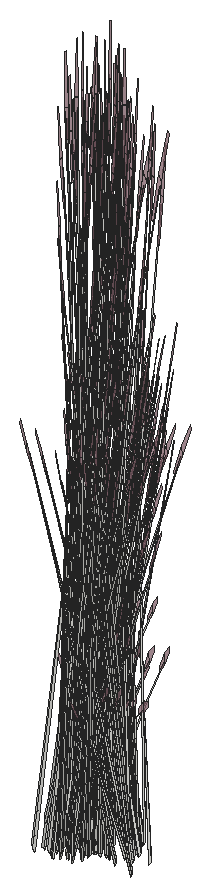
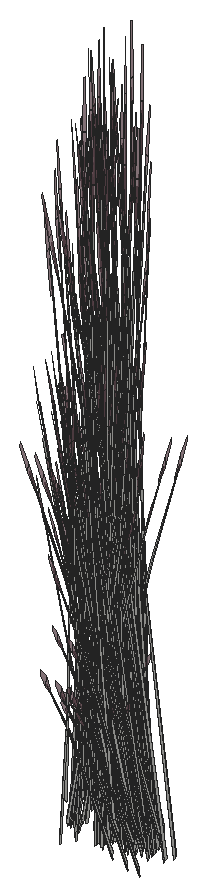
# SketchUp Ruby script. Lengths in inches.
U = 1.inch
M = Sketchup.active_model
def pt(a) = Geom::Point3d.new(a.map { |v| v * U })
def face(e, loops, mat)
  f = e.add_face(loops[0].map { |a| pt(a) })
  loops[1..].each { |l| e.add_face(l.map { |a| pt(a) }).erase! }
  f.material = f.back_material = mat if mat
  f
end
# faces: each face lists its corners as indices into pts; further lists are holes
def faces(e, pts, list, mat = nil) = list.each { |f| face(e, (f[0].is_a?(Array) ? f : [f]).map { |l| l.map { |i| pts[i] } }, mat) }
# xy, xz, yz: faces in a plane at the given z, y or x. An outline is a flat list of corners, or four numbers for a rectangle; further outlines are holes
def ring(l) = l.size == 4 ? [[l[0], l[1]], [l[2], l[1]], [l[2], l[3]], [l[0], l[3]]] : l.each_slice(2).to_a
def flat(e, list, mat, &to3) = list.each { |f| face(e, (f[0].is_a?(Array) ? f : [f]).map { |l| ring(l).map { |u, v| to3.(u, v) } }, mat) }
def xy(e, z, list, mat = nil) = flat(e, list, mat) { |x, y| [x, y, z] }
def xz(e, y, list, mat = nil) = flat(e, list, mat) { |x, z| [x, y, z] }
def yz(e, x, list, mat = nil) = flat(e, list, mat) { |y, z| [x, y, z] }
def lines(e, pts, list) = list.each { |a, b| e.add_line(pt(pts[a]), pt(pts[b])) }
# prism: a flat outline (further loops are holes) pulled along v
def prism(e, loops, v, mat = nil)
  f = face(e, loops, mat); d = Geom::Vector3d.new(v.map { |x| x * U })
  f.pushpull(f.normal.samedirection?(d) ? d.length : -d.length)
end
def box(e, o, s, mat = nil) = prism(e, [[o, [o[0] + s[0], o[1], o[2]], [o[0] + s[0], o[1] + s[1], o[2]], [o[0], o[1] + s[1], o[2]]]], [0, 0, s[2]], mat)
def at(x, y, z, deg = 0) = Geom::Transformation.translation(pt([x, y, z])) * Geom::Transformation.rotation(ORIGIN, Z_AXIS, deg.degrees)
def axes(o, x, y, z) = Geom::Transformation.new([*x, 0, *y, 0, *z, 0, *pt(o).to_a, 1])
def part(name) = M.definitions.add(name)
# library, detail: a bought-in or finely detailed component or shape, given as its bounding box
def library(name, o, s) = part(name).tap { |d| box(d.entities, o, s) }
def detail(e, o, s) = box(e.add_group.entities, o, s)
def put(e, d, t, mat = nil) = e.add_instance(d, t).tap { |i| i.material = mat if mat }
def group(e, t, mat = nil) = e.add_group.tap { |g| g.transformation = t; g.material = mat if mat }.entities
root = M.entities
M.materials.add("LightPink_Translucent").color = [144, 107, 117]
M.materials["LightPink_Translucent"].alpha = 0.75
c1 = part("blade")
p = [[2.15,0.21,22],[0,0.17,0],[0.09,0.45,0],[2.18,0.31,22],[2.29,0.31,22],[0.38,0.45,0],
  [2.48,0.24,33],[2.49,0.24,33],[2.48,0.22,33]]
faces(c1.entities,p,[[0,1,2,3],[4,5,2,3],[6,3,4,7],[8,0,3,6]])
c2 = part("seeds")
p = [[0.3,-0.1,1.38],[-0.01,-0.03,1.59],[-0.01,-0.03,0.03],[0.14,-0.07,-0.07],[0.29,-0.03,3],[0.15,0.01,3.11]]
faces(c2.entities,p,[[0,1,2,3],[1,0,4,5]],"LightPink_Translucent")
c3 = part("blade with seeds")
put(c3.entities,c1,at(0,0,0))
put(c3.entities,c2,axes([2.4,0.25,30.99],[1.5799,-0.05474,1.17369],[-0.12525,1.92788,0.29478],[-0.07173,-0.02425,1.56792]))
put(root,c3,axes([345.21,653.21,621.74],[-0.33032,0.23318,-0.49651],[-0.19744,-0.41812,0],[-0.07523,0.05311,1.57504]))
put(root,c3,axes([345.24,653.09,621.92],[-0.21791,-0.46895,-0.05142],[0.36918,-0.26061,0.51607],[-0.09097,0.04465,1.6363]))
put(root,c3,axes([341.87,652.99,624.37],[-0.05451,-0.37564,0.35414],[0.31161,-0.09919,-0.4572],[0.0837,0.10765,0.87481]))
put(root,c3,axes([341.6,652.74,623.95],[-0.01777,0.35463,0.0643],[-0.26836,-0.00972,0.50621],[0.1028,0.03711,0.77189]))
put(root,c3,axes([341.52,653.3,620.72],[0.02571,-0.06733,1.76342],[0.32373,-0.19829,-0.26939],[0.09815,0.10263,0.30037]))
put(root,c3,axes([341.62,652.63,623.96],[-0.26024,0.30729,0.48003],[-0.22444,-0.32634,0.3958],[0.1221,0.05668,0.9933]))
put(root,c3,axes([344.3,651.74,621.91],[-0.44111,-0.00373,-0.04976],[0,-0.52122,0.49943],[-0.01386,0.11865,1.58352]))
put(root,c3,axes([341.94,651.02,621.53],[0.21202,0.39143,-0.44739],[-0.32115,0.27564,0.21531],[0.06861,0.04843,1.43643]))
put(root,c3,axes([342.3,652.68,623.15],[-0.06755,-0.39203,-0.03492],[0.31928,-0.09013,-0.15832],[0.06667,0.02485,0.52218]))
put(root,c3,axes([345.14,653.03,621.75],[-0.32928,-0.11539,-0.30978],[0.08291,-0.40636,0.30978],[-0.06638,0.04686,1.38974]))
put(root,c3,axes([341.75,651.66,624.28],[-0.29332,-0.1301,0.35414],[0.08555,-0.37955,-0.4572],[0.11809,-0.0348,0.87481]))
put(root,c3,axes([343.43,650.18,622.18],[-0.37926,0.12378,0.17642],[-0.09365,-0.46065,0.35086],[0.03382,0.06712,1.60407]))
put(root,c3,axes([342.08,650.82,623.79],[-0.30498,-0.24231,1.38283],[0.32203,-0.37727,0.59665],[0.0984,0.22736,1.33663]))
put(root,c3,axes([343.73,652.64,624.78],[0.23881,-0.24554,0.35414],[0.22606,0.28036,-0.4572],[-0.0344,0.14245,0.87481]))
put(root,c3,axes([345.33,651.29,622.57],[-0.00964,-0.43909,1.41272],[0.43635,0.11382,0.59816],[-0.1032,0.24027,1.3335]))
put(root,c3,axes([341.57,653.51,624.03],[0.00104,-0.05646,1.77383],[0.30246,-0.2491,-0.16761],[0.10506,0.08891,0.31391]))
put(root,c3,axes([341.05,650.87,621.28],[0.36714,0.07646,-0.62353],[-0.07747,0.47163,-0.16365],[0.10956,0.05715,1.37633]))
put(root,c3,axes([342.54,652.8,622.08],[-0.19872,-0.13409,1.1486],[0.2566,-0.13625,0.84392],[0.06921,0.11541,0.25299]))
put(root,c3,axes([342.88,654.32,625.35],[0.2439,-0.26754,-0.06488],[0.22348,0.29302,-0.29416],[0.01573,0.08303,0.97024]))
put(root,c3,axes([341.84,652.65,621.91],[0.00623,-0.15459,1.43002],[0.29764,-0.17268,-0.30754],[0.09188,0.18503,0.61141]))
put(root,c3,axes([342.62,651.15,621.48],[-0.21881,-0.29821,-0.06488],[0.23965,-0.27324,-0.29416],[0.0679,-0.01924,0.97024]))
put(root,c3,axes([342.8125,650.85,622.07],[-0.29264,0.42323,0.45755],[-0.34767,-0.3736,0.17955],[0.07055,-0.04224,1.58856]))
put(root,c3,axes([347.2,650.8,624.1],[0.14639,-0.01056,1.71376],[-0.09712,0.45778,0.13857],[-0.20862,-0.02831,0.73262]))
put(root,c3,axes([343.3125,651.52,621.92],[0.24637,0.30123,0],[-0.24637,0.30123,0],[0,0,1.69266]))
put(root,c3,axes([343.3125,651.16,622.43],[0.17124,-0.42022,0.44739],[0.35581,0.20224,-0.21531],[0,0.09687,1.43643]))
put(root,c3,axes([343.16,652.62,621.91],[0.35581,0.20937,0],[-0.17124,0.43505,0],[0,0,1.74954]))
put(root,c3,axes([345.08,651.85,622.39],[0.04113,0.53214,-0.29095],[-0.42835,0.03218,-0.50002],[-0.07543,0.07088,1.59708]))
put(root,c3,axes([343.2,651.0625,622.09],[-0.44609,-0.09826,0.49198],[0.09078,-0.55493,0.19306],[0.06519,0.05359,1.70813]))
put(root,c3,axes([342.52,650.15,621.35],[0.08291,0.40636,-0.30978],[-0.32928,0.11539,0.30978],[0.06638,0.04686,1.38974]))
put(root,c3,axes([343.14,651.48,621.69],[0.44133,0,0],[0,0.52122,-0.51607],[0,0.11871,1.63711]))
put(root,c3,axes([344.21,651.82,621.74],[-0.24637,0.29097,-0.30978],[-0.24637,-0.29097,0.30978],[0,0.09372,1.38974]))
put(root,c3,axes([341.72,650.8,621.98],[0.35635,-0.30962,-0.29095],[0.23697,0.43749,-0.50002],[0.08792,0.04443,1.59708]))
put(root,c3,axes([343.51,651.77,621.8],[0.12941,0.42699,-0.69212],[-0.37279,0.15378,-0.18165],[0.0143,0.14459,1.52773]))
put(root,c3,axes([344.44,651.66,622.09],[0.44609,0.09826,0.45755],[-0.09078,0.55493,0.17955],[-0.06519,-0.05359,1.58856]))
put(root,c3,axes([343.32,651.31,621.91],[0.39487,0,0],[0,0.48281,0],[0,0,1.78407]))
put(root,c3,axes([342.57,653.41,621.98],[-0.22633,-0.01463,1.0506],[0.14947,-0.31064,0.58006],[0.08941,0.11036,0.8241]))
put(root,c3,axes([340.98,651.88,623.1],[-0.1311,-0.08035,1.71376],[0.27131,-0.33708,0.13857],[0.16909,0.15206,0.73262]))
put(root,c3,axes([342.94,650.78,622.43],[-0.21202,-0.39143,0.44739],[0.32115,-0.27564,-0.21531],[0.06861,0.04843,1.43643]))
put(root,c3,axes([343.46,651.26,622.32],[0.32884,-0.136,0.1448],[0.11516,0.38837,-0.41347],[0,0.08547,1.26744]))
put(root,c3,axes([347.26,651.61,624.1],[0.12246,-0.09864,1.71376],[0.1031,0.45582,0.13857],[-0.19225,0.10302,0.73262]))
put(root,c3,axes([344.33,651.55,622.44],[-0.17124,0.42022,0.44739],[-0.35581,-0.20224,-0.21531],[0,-0.09687,1.43643]))
put(root,c3,axes([342.01,651.78,623.95],[0.12963,0.31798,0.0643],[-0.23638,0.15564,0.50621],[0.1042,-0.03071,0.77189]))
put(root,c3,axes([341.7,652.63,623.75],[0.20082,0.29199,-0.35414],[-0.2293,0.2764,0.4572],[0.1165,0.04206,0.87481]))
put(root,c3,axes([346.875,652.38,622.82],[0.12266,0.03828,1.43002],[0.07906,0.39104,-0.30754],[-0.16661,0.0732,0.61141]))
put(root,c3,axes([341.47,652.66,624.26],[0.0189,-0.47427,-0.1216],[0.35781,0.01296,-0.67495],[0.13781,0.03295,1.02557]))
put(root,c3,axes([343.35,651.29,622.375],[0.39748,0.22252,-0.29095],[-0.19139,0.46966,-0.50002],[0.01249,0.11531,1.59708]))
put(root,c3,axes([341.99,651.66,623.96],[-0.09971,0.42522,0.48003],[-0.32782,-0.1454,0.3958],[0.12892,-0.02555,0.9933]))
put(root,c3,axes([341.84,653.18,624.35],[0.21031,-0.39918,-0.1216],[0.30457,0.22997,-0.67495],[0.10587,0.11278,1.02557]))
put(root,c3,axes([340.82,650.53,620.91],[-0.3474,0.18671,1.28929],[-0.11057,-0.53572,0.50096],[0.21332,0.00891,1.46642]))
put(root,c3,axes([344.2,652.54,622.2],[0.37926,-0.12378,0.17642],[0.09365,0.46065,0.35086],[-0.03382,-0.06712,1.60407]))
put(root,c3,axes([347.96,651.13,623.57],[0.10032,-0.06746,1.77064],[0.0346,0.47103,0.13857],[-0.2173,0.0625,0.63284]))
put(root,c3,axes([344.69,652.61,621.92],[-0.35581,-0.20937,0],[0.17124,-0.43505,0],[0,0,1.62707]))
put(root,c3,axes([345.51,653.14,622.1],[0.22066,0.46731,0],[-0.36918,0.26061,-0.51607],[-0.08408,0.05936,1.63711]))
put(root,c3,axes([344.21,651.4,622.1875],[0,-0.46636,0.49651],[0.39487,0,0],[0,0.10622,1.57504]))
put(root,c3,axes([344.38,651.83,621.72],[0,0.46636,-0.49651],[-0.39487,0,0],[0,0.10622,1.57504]))
put(root,c3,axes([343.32,653.24,624.44],[-0.35104,0.10702,0.48003],[-0.06092,-0.41983,0.3958],[0.08256,0.12373,0.9933]))
put(root,c3,axes([342.09,652.98,624],[0.34827,-0.11086,-0.51099],[0.06092,0.41983,-0.3958],[0.09354,0.12031,0.97773]))
put(root,c3,axes([343.26,653.33,624.4375],[-0.16041,0.29625,0.0643],[-0.22843,-0.17248,0.50621],[0.07385,0.09498,0.77189]))
put(root,c3,axes([343.09,650.67,622.32],[0.06809,-0.4162,0.1448],[0.33266,0.07225,-0.41347],[0.06054,0.04274,1.26744]))
put(root,c3,axes([342.49,652.48,624.37],[-0.20082,-0.29199,0.35414],[0.2293,-0.2764,-0.4572],[0.1165,0.04206,0.87481]))
put(root,c3,axes([341.78,652.38,623.9375],[0.07571,-0.00789,1.74944],[0.20767,-0.36231,-0.27667],[0.13467,0.04783,0.14031]))
put(root,c3,axes([345.33,652.57,622.2],[0.10196,-0.46348,0.17642],[0.3731,0.13116,0.35086],[-0.06445,0.00226,1.60407]))
put(root,c3,axes([345.16,651.95,622.34],[0.26075,0.2802,0.1448],[-0.2175,0.31612,-0.41347],[-0.06054,0.04274,1.26744]))
put(root,c3,axes([346.88,651.45,624.94],[-0.05763,0.06055,1.74944],[0.0049,0.44239,-0.27667],[-0.13211,0.05753,0.14031]))
put(root,c3,axes([342.61,649.98,621.33],[0.33032,0.23318,-0.49651],[-0.19744,0.41812,0],[0.07523,0.05311,1.57504]))
put(root,c3,axes([345.07,651.61,622.02],[-0.32829,-0.4014,-0.06131],[0.32849,-0.40164,0],[-0.01146,-0.01402,1.75571]))
put(root,c3,axes([342.68,652.74,624.05],[-0.01777,0.35463,0.0643],[-0.26836,-0.00972,0.50621],[0.1028,0.03711,0.77189]))
put(root,c3,axes([345.15,651.75,622.44],[0.38326,-0.02879,0.44739],[0.03466,0.47788,-0.21531],[-0.06861,0.04843,1.43643]))
put(root,c3,axes([342.68,651.7,621.99],[-0.21807,0.07699,1.1486],[0.10265,-0.31819,0.84392],[0.11568,0.02177,0.25299]))
put(root,c3,axes([342.6,653.3,620.81],[0.02571,-0.06733,1.76342],[0.32373,-0.19829,-0.26939],[0.09815,0.10263,0.30037]))
put(root,c3,axes([343.56,649.94,622.1875],[-0.33032,-0.23318,0.49651],[0.19744,-0.41812,0],[0.07523,0.05311,1.57504]))
put(root,c3,axes([342.7,652.63,624.05],[-0.26024,0.30729,0.48003],[-0.22444,-0.32634,0.3958],[0.1221,0.05668,0.9933]))
put(root,c3,axes([347.07,651.19,624.75],[-0.29332,-0.1301,-0.35414],[0.08555,-0.37955,0.4572],[-0.11809,0.0348,0.87481]))
put(root,c3,axes([345.25,652.85,622.06],[0.44186,0.15158,0.30756],[-0.11054,0.54181,-0.36492],[-0.07313,0.06781,1.64885]))
put(root,c3,axes([343.375,652.68,623.25],[-0.06755,-0.39203,-0.03492],[0.31928,-0.09013,-0.15832],[0.06667,0.02485,0.52218]))
put(root,c3,axes([342.82,651.66,624.37],[-0.29332,-0.1301,0.35414],[0.08555,-0.37955,-0.4572],[0.11809,-0.0348,0.87481]))
put(root,c3,axes([343.27,652.375,621.89],[0.37054,-0.15823,-0.19198],[0.1302,0.45581,0.00008],[0.0409,-0.01749,1.73897]))
put(root,c3,axes([345.4375,652.82,622.2],[0.33032,-0.23318,0.49651],[0.19744,0.41812,0],[-0.07523,0.05311,1.57504]))
put(root,c3,axes([342.05,651.62,623.75],[0.29332,0.1301,-0.35414],[-0.08555,0.37955,0.4572],[0.11809,-0.0348,0.87481]))
put(root,c3,axes([342.13,650.87,621.375],[0.36714,0.07646,-0.62353],[-0.07747,0.47163,-0.16365],[0.10956,0.05715,1.37633]))
put(root,c3,axes([343.7,651.15,621.58],[-0.21881,-0.29821,-0.06488],[0.23965,-0.27324,-0.29416],[0.0679,-0.01924,0.97024]))
put(root,c3,axes([346.24,651.89,624.93],[0.04504,0.01251,1.77383],[0.13934,0.41205,-0.16761],[-0.0922,0.10815,0.31391]))
put(root,c3,axes([347.27,651.39,624.91],[-0.09562,0.42421,-0.51099],[-0.32782,-0.1454,-0.3958],[-0.13199,0.0389,0.97773]))
put(root,c3,axes([344.77,652.43,621.93],[-0.11516,-0.40207,0],[0.32884,-0.1408,0],[0,0,1.54371]))
put(root,c3,axes([341.49,652.4375,624.21],[0.35281,0.01123,-0.71045],[-0.0237,0.47284,0.08574],[0.14947,0.0499,1.00501]))
put(root,c3,axes([343.21,652.99,624.76],[-0.05451,-0.37564,0.35414],[0.31161,-0.09919,-0.4572],[0.0837,0.10765,0.87481]))
put(root,c3,axes([342.2,651.54,621.21],[-0.22732,0.05597,1.41583],[-0.03618,-0.44548,0.08104],[0.15921,-0.06743,0.80566]))
put(root,c3,axes([343.28,651.02,621.92],[0.21202,0.39143,-0.44739],[-0.32115,0.27564,0.21531],[0.06861,0.04843,1.43643]))
put(root,c3,axes([347.11,651.36,621.72],[0.00895,0.0735,1.76342],[-0.18044,0.38382,-0.26939],[-0.12817,-0.01935,0.30037]))
put(root,c3,axes([342.45,651.25,620.72],[-0.01845,-0.0708,1.76342],[0.12793,-0.41416,-0.26939],[0.12905,-0.00596,0.30037]))
put(root,c3,axes([348.39,651.04,623.57],[0.14639,-0.01056,1.71376],[-0.09712,0.45778,0.13857],[-0.20862,-0.02831,0.73262]))
put(root,c3,axes([342.58,653.04,623.93],[-0.03191,-0.04083,1.77383],[0.06981,-0.43764,-0.16761],[0.12571,-0.02796,0.31391]))
put(root,c3,axes([343.42,650.82,624.18],[-0.30498,-0.24231,1.38283],[0.32203,-0.37727,0.59665],[0.0984,0.22736,1.33663]))
put(root,c3,axes([341.26,651.15,623.1],[-0.14639,0.01056,1.71376],[0.09712,-0.45778,0.13857],[0.20862,0.02831,0.73262]))
put(root,c3,axes([342.9,653.51,624.42],[0.00104,-0.05646,1.77383],[0.30246,-0.2491,-0.16761],[0.10506,0.08891,0.31391]))
put(root,c3,axes([343.88,652.8,622.47],[-0.19872,-0.13409,1.1486],[0.2566,-0.13625,0.84392],[0.06921,0.11541,0.25299]))
put(root,c3,axes([345.24,651.64,621.9375],[-0.17124,0.42022,-0.44739],[-0.35581,-0.20224,0.21531],[0,0.09687,1.43643]))
put(root,c3,axes([346.62,653.2,622.99],[0.14709,-0.21136,1.1486],[0.05804,0.3346,0.84392],[-0.1063,0.05991,0.25299]))
put(root,c3,axes([342.06,651.88,623.19],[-0.1311,-0.08035,1.71376],[0.27131,-0.33708,0.13857],[0.16909,0.15206,0.73262]))
put(root,c3,axes([341.79,651.58,624.21],[0.31014,-0.20596,-0.71045],[0.17284,0.42397,0.08574],[0.14985,-0.04816,1.00501]))
put(root,c3,axes([347.14,651.15,624.96],[0.09971,-0.42522,0.48003],[0.32782,0.1454,0.3958],[-0.12892,0.02555,0.9933]))
put(root,c3,axes([345.91,651.38,622.2],[-0.2773,-0.3397,0.17642],[0.27945,-0.32949,0.35086],[-0.03063,0.06937,1.60407]))
put(root,c3,axes([347.25,651.02,625.26],[0.17758,0.42229,-0.1216],[-0.31518,0.20752,-0.67495],[-0.13282,0.05572,1.02557]))
put(root,c3,axes([344.96,651.1875,621.93],[0,-0.53961,0],[0.44133,0,0],[0,0,1.79456]))
put(root,c3,axes([347.11,651.03,624.96],[-0.12963,-0.31798,0.0643],[0.23638,-0.15564,0.50621],[-0.1042,0.03071,0.77189]))
put(root,c3,axes([345.18,651.4,622.02],[0,0.53934,-0.05637],[-0.44133,0,0],[0,0.01695,1.79368]))
put(root,c3,axes([343.86,650.15,621.74],[0.08291,0.40636,-0.30978],[-0.32928,0.11539,0.30978],[0.06638,0.04686,1.38974]))
put(root,c3,axes([344.48,651.48,622.08],[0.44133,0,0],[0,0.52122,-0.51607],[0,0.11871,1.63711]))
put(root,c3,axes([343.09,651.78,624.05],[0.12963,0.31798,0.0643],[-0.23638,0.15564,0.50621],[0.1042,-0.03071,0.77189]))
put(root,c3,axes([347.71,651.91,624.1],[0.08815,-0.14329,1.71376],[0.22258,0.38678,0.13857],[-0.15267,0.17614,0.73262]))
put(root,c3,axes([347.18,652.29,624.75],[-0.30722,0.06665,-0.35414],[-0.08112,-0.381,0.4572],[-0.08804,0.10234,0.87481]))
put(root,c3,axes([344.4,653.05,624.78],[0.1064,-0.35863,0.35414],[0.31043,0.1046,-0.4572],[0.02846,0.14439,0.87481]))
put(root,c3,axes([342.78,652.63,623.84],[0.20082,0.29199,-0.35414],[-0.2293,0.2764,0.4572],[0.1165,0.04206,0.87481]))
put(root,c3,axes([342.55,652.66,624.35],[0.0189,-0.47427,-0.1216],[0.35781,0.01296,-0.67495],[0.13781,0.03295,1.02557]))
put(root,c3,axes([348.45,651.84,623.57],[0.12246,-0.09864,1.71376],[0.1031,0.45582,0.13857],[-0.19225,0.10302,0.73262]))
put(root,c3,axes([344.24,650.15,622.2],[-0.10196,0.46348,0.17642],[-0.3731,-0.13116,0.35086],[0.06445,-0.00226,1.60407]))
put(root,c3,axes([343.06,651.66,624.05],[-0.09971,0.42522,0.48003],[-0.32782,-0.1454,0.3958],[0.12892,-0.02555,0.9933]))
put(root,c3,axes([347.01,653.42,621.72],[0.04734,0.04659,1.76342],[0.08027,0.4317,-0.26939],[-0.10492,0.09206,0.30037]))
put(root,c3,axes([344.97,652.45,622.02],[0.15345,0.53576,-0.06012],[-0.43845,0.18773,0],[0.00536,0.01871,1.72173]))
put(root,c3,axes([343.05,650.8,622.375],[0.35635,-0.30962,-0.29095],[0.23697,0.43749,-0.50002],[0.08792,0.04443,1.59708]))
put(root,c3,axes([343.91,653.41,622.375],[-0.22633,-0.01463,1.0506],[0.14947,-0.31064,0.58006],[0.08941,0.11036,0.8241]))
put(root,c3,axes([348.07,652.62,622.28],[0.12266,0.03828,1.43002],[0.07906,0.39104,-0.30754],[-0.16661,0.0732,0.61141]))
put(root,c3,axes([342.27,652.21,621.81],[-0.085,-0.1147,1.43002],[0.1106,-0.37943,-0.30754],[0.17198,0.0514,0.61141]))
put(root,c3,axes([347.22,652.2,624.96],[-0.08753,-0.42921,0.48003],[0.34336,-0.07449,0.3958],[-0.1012,0.10094,0.9933]))
put(root,c3,axes([346.23,651.74,621.93],[-0.44111,-0.00373,-0.04976],[0,-0.52122,0.49943],[-0.01386,0.11865,1.58352]))
put(root,c3,axes([349.16,651.37,623.03],[0.10032,-0.06746,1.77064],[0.0346,0.47103,0.13857],[-0.2173,0.0625,0.63284]))
put(root,c3,axes([345.37,650.18,622.2],[-0.37926,0.12378,0.17642],[-0.09365,-0.46065,0.35086],[0.03382,0.06712,1.60407]))
put(root,c3,axes([347.15,652.12,624.96],[-0.2423,-0.19613,0.0643],[0.14107,-0.2793,0.50621],[-0.07768,0.0903,0.77189]))
put(root,c3,axes([342.86,652.38,624.03],[0.07571,-0.00789,1.74944],[0.20767,-0.36231,-0.27667],[0.13467,0.04783,0.14031]))
put(root,c3,axes([343.18,653.18,624.74],[0.21031,-0.39918,-0.1216],[0.30457,0.22997,-0.67495],[0.10587,0.11278,1.02557]))
put(root,c3,axes([342.15,650.53,621.3],[-0.3474,0.18671,1.28929],[-0.11057,-0.53572,0.50096],[0.21332,0.00891,1.46642]))
put(root,c3,axes([344.8125,654.32,625.37],[0.2439,-0.26754,-0.06488],[0.22348,0.29302,-0.29416],[0.01573,0.08303,0.97024]))
put(root,c3,axes([344.75,650.85,622.09],[-0.29264,0.42323,0.45755],[-0.34767,-0.3736,0.17955],[0.07055,-0.04224,1.58856]))
put(root,c3,axes([345.25,651.52,621.94],[0.24637,0.30123,0],[-0.24637,0.30123,0],[0,0,1.69266]))
put(root,c3,axes([343.76,651.7,622.08],[-0.21807,0.07699,1.1486],[0.10265,-0.31819,0.84392],[0.11568,0.02177,0.25299]))
put(root,c3,axes([345.24,651.16,622.44],[0.17124,-0.42022,0.44739],[0.35581,0.20224,-0.21531],[0,0.09687,1.43643]))
put(root,c3,axes([345.1,652.62,621.93],[0.35581,0.20937,0],[-0.17124,0.43505,0],[0,0,1.74954]))
put(root,c3,axes([348.08,651.68,624.41],[-0.05763,0.06055,1.74944],[0.0049,0.44239,-0.27667],[-0.13211,0.05753,0.14031]))
put(root,c3,axes([343.43,652.98,624.39],[0.34827,-0.11086,-0.51099],[0.06092,0.41983,-0.3958],[0.09354,0.12031,0.97773]))
put(root,c3,axes([347.38,651.15,625.28],[0.29332,0.1301,0.35414],[-0.08555,0.37955,-0.4572],[-0.11809,0.0348,0.87481]))
put(root,c3,axes([343.13,651.62,623.84],[0.29332,0.1301,-0.35414],[-0.08555,0.37955,0.4572],[0.11809,-0.0348,0.87481]))
put(root,c3,axes([345.13,651.0625,622.11],[-0.44609,-0.09826,0.49198],[0.09078,-0.55493,0.19306],[0.06519,0.05359,1.70813]))
put(root,c3,axes([343.83,652.48,624.76],[-0.20082,-0.29199,0.35414],[0.2293,-0.2764,-0.4572],[0.1165,0.04206,0.87481]))
put(root,c3,axes([347.43,652.33,624.91],[0.09067,0.42583,-0.51099],[-0.34336,0.07449,-0.3958],[-0.0984,0.11438,0.97773]))
put(root,c3,axes([348.26,651.43,624.22],[-0.29332,-0.1301,-0.35414],[0.08555,-0.37955,0.4572],[-0.11809,0.0348,0.87481]))
put(root,c3,axes([346.14,651.82,621.75],[-0.24637,0.29097,-0.30978],[-0.24637,-0.29097,0.30978],[0,0.09372,1.38974]))
put(root,c3,axes([343.95,649.98,621.72],[0.33032,0.23318,-0.49651],[-0.19744,0.41812,0],[0.07523,0.05311,1.57504]))
put(root,c3,axes([342.57,652.4375,624.3],[0.35281,0.01123,-0.71045],[-0.0237,0.47284,0.08574],[0.14947,0.0499,1.00501]))
put(root,c3,axes([348.29,652.03,622.28],[-0.36714,-0.07646,-0.62353],[0.07747,-0.47163,-0.16365],[-0.10956,-0.05715,1.37633]))
put(root,c3,axes([344.01,652.74,624.4375],[-0.01777,0.35463,0.0643],[-0.26836,-0.00972,0.50621],[0.1028,0.03711,0.77189]))
put(root,c3,axes([345.4375,651.77,621.82],[0.12941,0.42699,-0.69212],[-0.37279,0.15378,-0.18165],[0.0143,0.14459,1.52773]))
put(root,c3,axes([343.93,653.3,621.2],[0.02571,-0.06733,1.76342],[0.32373,-0.19829,-0.26939],[0.09815,0.10263,0.30037]))
put(root,c3,axes([344.04,652.63,624.44],[-0.26024,0.30729,0.48003],[-0.22444,-0.32634,0.3958],[0.1221,0.05668,0.9933]))
put(root,c3,axes([345.26,651.31,621.93],[0.39487,0,0],[0,0.48281,0],[0,0,1.78407]))
put(root,c3,axes([343.28,651.54,621.3],[-0.22732,0.05597,1.41583],[-0.03618,-0.44548,0.08104],[0.15921,-0.06743,0.80566]))
put(root,c3,axes([347.4375,652.13,624.4],[0.04504,0.01251,1.77383],[0.13934,0.41205,-0.16761],[-0.0922,0.10815,0.31391]))
put(root,c3,axes([343.53,651.25,620.81],[-0.01845,-0.0708,1.76342],[0.12793,-0.41416,-0.26939],[0.12905,-0.00596,0.30037]))
put(root,c3,axes([348.46,651.625,624.37],[-0.09562,0.42421,-0.51099],[-0.32782,-0.1454,-0.3958],[-0.13199,0.0389,0.97773]))
put(root,c3,axes([344.875,650.78,622.44],[-0.21202,-0.39143,0.44739],[0.32115,-0.27564,-0.21531],[0.06861,0.04843,1.43643]))
put(root,c3,axes([344.71,652.68,623.64],[-0.06755,-0.39203,-0.03492],[0.31928,-0.09013,-0.15832],[0.06667,0.02485,0.52218]))
put(root,c3,axes([345.39,651.26,622.34],[0.32884,-0.136,0.1448],[0.11516,0.38837,-0.41347],[0,0.08547,1.26744]))
put(root,c3,axes([344.16,651.66,624.76],[-0.29332,-0.1301,0.35414],[0.08555,-0.37955,-0.4572],[0.11809,-0.0348,0.87481]))
put(root,c3,axes([343.65,653.04,624.03],[-0.03191,-0.04083,1.77383],[0.06981,-0.43764,-0.16761],[0.12571,-0.02796,0.31391]))
put(root,c3,axes([342.33,651.15,623.19],[-0.14639,0.01056,1.71376],[0.09712,-0.45778,0.13857],[0.20862,0.02831,0.73262]))
put(root,c3,axes([348.3,651.6,621.18],[0.00895,0.0735,1.76342],[-0.18044,0.38382,-0.26939],[-0.12817,-0.01935,0.30037]))
put(root,c3,axes([343.47,650.87,621.77],[0.36714,0.07646,-0.62353],[-0.07747,0.47163,-0.16365],[0.10956,0.05715,1.37633]))
put(root,c3,axes([345.03,651.15,621.97],[-0.21881,-0.29821,-0.06488],[0.23965,-0.27324,-0.29416],[0.0679,-0.01924,0.97024]))
put(root,c3,axes([347.8,652.92,622.24],[-0.33032,-0.23318,-0.49651],[0.19744,-0.41812,0],[-0.07523,-0.05311,1.57504]))
put(root,c3,axes([347.27,652.03,625.26],[0.32648,0.25715,-0.1216],[-0.18809,0.3724,-0.67495],[-0.09224,0.12945,1.02557]))
put(root,c3,axes([345.28,651.29,622.39],[0.39748,0.22252,-0.29095],[-0.19139,0.46966,-0.50002],[0.01249,0.11531,1.59708]))
put(root,c3,axes([342.87,651.58,624.3],[0.31014,-0.20596,-0.71045],[0.17284,0.42397,0.08574],[0.14985,-0.04816,1.00501]))
put(root,c3,axes([348,653.2,622.6],[-0.22066,0.46731,0],[-0.36918,-0.26061,-0.51607],[-0.08408,-0.05936,1.63711]))
put(root,c3,axes([347.82,653.4375,622.46],[0.14709,-0.21136,1.1486],[0.05804,0.3346,0.84392],[-0.1063,0.05991,0.25299]))
put(root,c3,axes([348.33,651.38,624.42],[0.09971,-0.42522,0.48003],[0.32782,0.1454,0.3958],[-0.12892,0.02555,0.9933]))
put(root,c3,axes([346.14,651.4,622.2],[0,-0.46636,0.49651],[0.39487,0,0],[0,0.10622,1.57504]))
put(root,c3,axes([346.3125,651.83,621.74],[0,0.46636,-0.49651],[-0.39487,0,0],[0,0.10622,1.57504]))
put(root,c3,axes([345.26,653.24,624.46],[-0.35104,0.10702,0.48003],[-0.06092,-0.41983,0.3958],[0.08256,0.12373,0.9933]))
put(root,c3,axes([348.45,651.26,624.73],[0.17758,0.42229,-0.1216],[-0.31518,0.20752,-0.67495],[-0.13282,0.05572,1.02557]))
put(root,c3,axes([346.73,653.14,625.87],[0.31145,0.12449,-0.06488],[-0.0958,0.38314,-0.29416],[-0.05094,0.05817,0.97024]))
put(root,c3,axes([345.19,653.33,624.46],[-0.16041,0.29625,0.0643],[-0.22843,-0.17248,0.50621],[0.07385,0.09498,0.77189]))
put(root,c3,axes([348.85,650.38,624.73],[-0.0189,0.47427,-0.1216],[-0.35781,-0.01296,-0.67495],[-0.13781,-0.03295,1.02557]))
put(root,c3,axes([348.31,651.27,624.42],[-0.12963,-0.31798,0.0643],[0.23638,-0.15564,0.50621],[-0.1042,0.03071,0.77189]))
put(root,c3,axes([345.02,650.67,622.34],[0.06809,-0.4162,0.1448],[0.33266,0.07225,-0.41347],[0.06054,0.04274,1.26744]))
put(root,c3,axes([347.43,652.0625,625.28],[0.30722,-0.06665,0.35414],[0.08112,0.381,-0.4572],[-0.08804,0.10234,0.87481]))
put(root,c3,axes([348.9,652.15,623.57],[0.08815,-0.14329,1.71376],[0.22258,0.38678,0.13857],[-0.15267,0.17614,0.73262]))
put(root,c3,axes([348.37,652.52,624.22],[-0.30722,0.06665,-0.35414],[-0.08112,-0.381,0.4572],[-0.08804,0.10234,0.87481]))
put(root,c3,axes([343.39,651.88,623.58],[-0.1311,-0.08035,1.71376],[0.27131,-0.33708,0.13857],[0.16909,0.15206,0.73262]))
put(root,c3,axes([343.35,652.21,621.91],[-0.085,-0.1147,1.43002],[0.1106,-0.37943,-0.30754],[0.17198,0.0514,0.61141]))
put(root,c3,axes([348.2,653.66,621.18],[0.04734,0.04659,1.76342],[0.08027,0.4317,-0.26939],[-0.10492,0.09206,0.30037]))
put(root,c3,axes([348.13,651.12,622.46],[0.22533,-0.03337,1.1486],[-0.14293,0.29403,0.84392],[-0.11135,-0.04411,0.25299]))
put(root,c3,axes([345.49,649.94,622.2],[-0.33032,-0.23318,0.49651],[0.19744,-0.41812,0],[0.07523,0.05311,1.57504]))
put(root,c3,axes([344.42,651.78,624.4375],[0.12963,0.31798,0.0643],[-0.23638,0.15564,0.50621],[0.1042,-0.03071,0.77189]))
put(root,c3,axes([344.11,652.63,624.23],[0.20082,0.29199,-0.35414],[-0.2293,0.2764,0.4572],[0.1165,0.04206,0.87481]))
put(root,c3,axes([343.88,652.66,624.74],[0.0189,-0.47427,-0.1216],[0.35781,0.01296,-0.67495],[0.13781,0.03295,1.02557]))
put(root,c3,axes([345.2,652.375,621.91],[0.37054,-0.15823,-0.19198],[0.1302,0.45581,0.00008],[0.0409,-0.01749,1.73897]))
